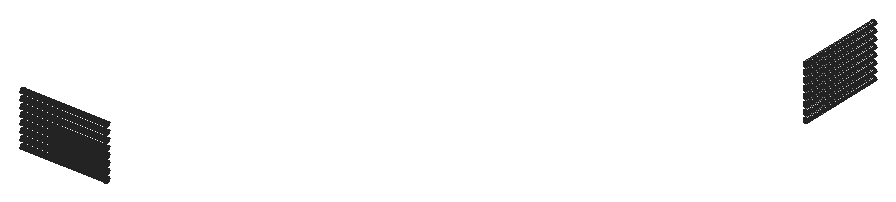
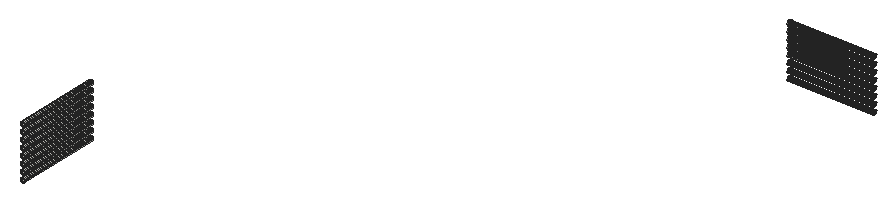
# SketchUp Ruby script. Lengths in inches.
U = 1.inch
M = Sketchup.active_model
def pt(a) = Geom::Point3d.new(a.map { |v| v * U })
def face(e, loops, mat)
  f = e.add_face(loops[0].map { |a| pt(a) })
  loops[1..].each { |l| e.add_face(l.map { |a| pt(a) }).erase! }
  f.material = f.back_material = mat if mat
  f
end
# faces: each face lists its corners as indices into pts; further lists are holes
def faces(e, pts, list, mat = nil) = list.each { |f| face(e, (f[0].is_a?(Array) ? f : [f]).map { |l| l.map { |i| pts[i] } }, mat) }
# xy, xz, yz: faces in a plane at the given z, y or x. An outline is a flat list of corners, or four numbers for a rectangle; further outlines are holes
def ring(l) = l.size == 4 ? [[l[0], l[1]], [l[2], l[1]], [l[2], l[3]], [l[0], l[3]]] : l.each_slice(2).to_a
def flat(e, list, mat, &to3) = list.each { |f| face(e, (f[0].is_a?(Array) ? f : [f]).map { |l| ring(l).map { |u, v| to3.(u, v) } }, mat) }
def xy(e, z, list, mat = nil) = flat(e, list, mat) { |x, y| [x, y, z] }
def xz(e, y, list, mat = nil) = flat(e, list, mat) { |x, z| [x, y, z] }
def yz(e, x, list, mat = nil) = flat(e, list, mat) { |y, z| [x, y, z] }
def lines(e, pts, list) = list.each { |a, b| e.add_line(pt(pts[a]), pt(pts[b])) }
# prism: a flat outline (further loops are holes) pulled along v
def prism(e, loops, v, mat = nil)
  f = face(e, loops, mat); d = Geom::Vector3d.new(v.map { |x| x * U })
  f.pushpull(f.normal.samedirection?(d) ? d.length : -d.length)
end
def box(e, o, s, mat = nil) = prism(e, [[o, [o[0] + s[0], o[1], o[2]], [o[0] + s[0], o[1] + s[1], o[2]], [o[0], o[1] + s[1], o[2]]]], [0, 0, s[2]], mat)
def at(x, y, z, deg = 0) = Geom::Transformation.translation(pt([x, y, z])) * Geom::Transformation.rotation(ORIGIN, Z_AXIS, deg.degrees)
def axes(o, x, y, z) = Geom::Transformation.new([*x, 0, *y, 0, *z, 0, *pt(o).to_a, 1])
def part(name) = M.definitions.add(name)
# library, detail: a bought-in or finely detailed component or shape, given as its bounding box
def library(name, o, s) = part(name).tap { |d| box(d.entities, o, s) }
def detail(e, o, s) = box(e.add_group.entities, o, s)
def put(e, d, t, mat = nil) = e.add_instance(d, t).tap { |i| i.material = mat if mat }
def group(e, t, mat = nil) = e.add_group.tap { |g| g.transformation = t; g.material = mat if mat }.entities
root = M.entities
p = [[922.01,48.34,1629.02],[922.01,47.38,1629.14],[778.64,47.38,1629.14],[778.64,48.34,1629.02],[922.01,49.29,1629.14],[778.64,49.29,1629.14],
  [1535.52,886.83,1629.14],[1536.47,886.83,1629.02],[1536.47,743.45,1629.02],[1535.52,743.45,1629.14],[1537.43,886.83,1629.14],[1537.43,743.45,1629.14],
  [922.01,46.5,1629.51],[778.64,46.5,1629.51],[922.01,50.18,1629.51],[778.64,50.18,1629.51],[1534.63,886.83,1629.51],[1534.63,743.45,1629.51],
  [1538.32,886.83,1629.51],[1538.32,743.45,1629.51],[922.01,45.73,1630.1],[778.64,45.73,1630.1],[922.01,50.95,1630.1],[778.64,50.95,1630.1],
  [1533.87,886.83,1630.1],[1533.87,743.45,1630.1],[1539.08,886.83,1630.1],[1539.08,743.45,1630.1],[922.01,45.15,1630.86],[778.64,45.15,1630.86],
  [922.01,51.53,1630.86],[778.64,51.53,1630.86],[1533.28,886.83,1630.86],[1533.28,743.45,1630.86],[1539.67,886.83,1630.86],[1539.67,743.45,1630.86],
  [922.01,44.78,1631.75],[778.64,44.78,1631.75],[922.01,51.9,1631.75],[778.64,51.9,1631.75],[1532.91,886.83,1631.75],[1532.91,743.45,1631.75],
  [1540.03,886.83,1631.75],[1540.03,743.45,1631.75],[922.01,44.65,1632.7],[778.64,44.65,1632.7],[922.01,52.03,1632.7],[778.64,52.03,1632.7],
  [1532.79,886.83,1632.7],[1532.79,743.45,1632.7],[1540.16,886.83,1632.7],[1540.16,743.45,1632.7],[922.01,44.78,1633.66],[778.64,44.78,1633.66],
  [922.01,51.9,1633.66],[778.64,51.9,1633.66],[1532.91,886.83,1633.66],[1532.91,743.45,1633.66],[1540.03,886.83,1633.66],[1540.03,743.45,1633.66],
  [922.01,45.15,1634.55],[778.64,45.15,1634.55],[922.01,51.53,1634.55],[778.64,51.53,1634.55],[1533.28,886.83,1634.55],[1533.28,743.45,1634.55],
  [1539.67,886.83,1634.55],[1539.67,743.45,1634.55],[922.01,45.73,1635.3125],[778.64,45.73,1635.3125],[922.01,50.95,1635.3125],[778.64,50.95,1635.3125],
  [1533.87,886.83,1635.3125],[1533.87,743.45,1635.3125],[1539.08,886.83,1635.3125],[1539.08,743.45,1635.3125],[922.01,46.5,1635.9],[778.64,46.5,1635.9],
  [922.01,50.18,1635.9],[778.64,50.18,1635.9],[1534.63,886.83,1635.9],[1534.63,743.45,1635.9],[1538.32,886.83,1635.9],[1538.32,743.45,1635.9],
  [922.01,47.38,1636.27],[778.64,47.38,1636.27],[922.01,49.29,1636.27],[778.64,49.29,1636.27],[1535.52,886.83,1636.27],[1535.52,743.45,1636.27],
  [1537.43,886.83,1636.27],[1537.43,743.45,1636.27],[922.01,48.34,1636.39],[778.64,48.34,1636.39],[1536.47,886.83,1636.39],[1536.47,743.45,1636.39],
  [922.01,48.34,1641.02],[922.01,47.38,1641.14],[778.64,47.38,1641.14],[778.64,48.34,1641.02],[922.01,49.29,1641.14],[778.64,49.29,1641.14],
  [1535.52,886.83,1641.14],[1536.47,886.83,1641.02],[1536.47,743.45,1641.02],[1535.52,743.45,1641.14],[1537.43,886.83,1641.14],[1537.43,743.45,1641.14],
  [922.01,46.5,1641.51],[778.64,46.5,1641.51],[922.01,50.18,1641.51],[778.64,50.18,1641.51],[1534.63,886.83,1641.51],[1534.63,743.45,1641.51],
  [1538.32,886.83,1641.51],[1538.32,743.45,1641.51],[922.01,45.73,1642.1],[778.64,45.73,1642.1],[922.01,50.95,1642.1],[778.64,50.95,1642.1],
  [1533.87,886.83,1642.1],[1533.87,743.45,1642.1],[1539.08,886.83,1642.1],[1539.08,743.45,1642.1],[922.01,45.15,1642.86],[778.64,45.15,1642.86],
  [922.01,51.53,1642.86],[778.64,51.53,1642.86],[1533.28,886.83,1642.86],[1533.28,743.45,1642.86],[1539.67,886.83,1642.86],[1539.67,743.45,1642.86],
  [922.01,44.78,1643.75],[778.64,44.78,1643.75],[922.01,51.9,1643.75],[778.64,51.9,1643.75],[1532.91,886.83,1643.75],[1532.91,743.45,1643.75],
  [1540.03,886.83,1643.75],[1540.03,743.45,1643.75],[922.01,44.65,1644.7],[778.64,44.65,1644.7],[922.01,52.03,1644.7],[778.64,52.03,1644.7],
  [1532.79,886.83,1644.7],[1532.79,743.45,1644.7],[1540.16,886.83,1644.7],[1540.16,743.45,1644.7],[922.01,44.78,1645.66],[778.64,44.78,1645.66],
  [922.01,51.9,1645.66],[778.64,51.9,1645.66],[1532.91,886.83,1645.66],[1532.91,743.45,1645.66],[1540.03,886.83,1645.66],[1540.03,743.45,1645.66],
  [922.01,45.15,1646.55],[778.64,45.15,1646.55],[922.01,51.53,1646.55],[778.64,51.53,1646.55],[1533.28,886.83,1646.55],[1533.28,743.45,1646.55],
  [1539.67,886.83,1646.55],[1539.67,743.45,1646.55],[922.01,45.73,1647.3125],[778.64,45.73,1647.3125],[922.01,50.95,1647.3125],[778.64,50.95,1647.3125],
  [1533.87,886.83,1647.3125],[1533.87,743.45,1647.3125],[1539.08,886.83,1647.3125],[1539.08,743.45,1647.3125],[922.01,46.5,1647.9],[778.64,46.5,1647.9],
  [922.01,50.18,1647.9],[778.64,50.18,1647.9],[1534.63,886.83,1647.9],[1534.63,743.45,1647.9],[1538.32,886.83,1647.9],[1538.32,743.45,1647.9],
  [922.01,47.38,1648.27],[778.64,47.38,1648.27],[922.01,49.29,1648.27],[778.64,49.29,1648.27],[1535.52,886.83,1648.27],[1535.52,743.45,1648.27],
  [1537.43,886.83,1648.27],[1537.43,743.45,1648.27],[922.01,48.34,1648.39],[778.64,48.34,1648.39],[1536.47,886.83,1648.39],[1536.47,743.45,1648.39],
  [922.01,48.34,1653.02],[922.01,47.38,1653.14],[778.64,47.38,1653.14],[778.64,48.34,1653.02],[922.01,49.29,1653.14],[778.64,49.29,1653.14],
  [1535.52,886.83,1653.14],[1536.47,886.83,1653.02],[1536.47,743.45,1653.02],[1535.52,743.45,1653.14],[1537.43,886.83,1653.14],[1537.43,743.45,1653.14],
  [922.01,46.5,1653.51],[778.64,46.5,1653.51],[922.01,50.18,1653.51],[778.64,50.18,1653.51],[1534.63,886.83,1653.51],[1534.63,743.45,1653.51],
  [1538.32,886.83,1653.51],[1538.32,743.45,1653.51],[922.01,45.73,1654.1],[778.64,45.73,1654.1],[922.01,50.95,1654.1],[778.64,50.95,1654.1],
  [1533.87,886.83,1654.1],[1533.87,743.45,1654.1],[1539.08,886.83,1654.1],[1539.08,743.45,1654.1],[922.01,45.15,1654.86],[778.64,45.15,1654.86],
  [922.01,51.53,1654.86],[778.64,51.53,1654.86],[1533.28,886.83,1654.86],[1533.28,743.45,1654.86],[1539.67,886.83,1654.86],[1539.67,743.45,1654.86],
  [922.01,44.78,1655.75],[778.64,44.78,1655.75],[922.01,51.9,1655.75],[778.64,51.9,1655.75],[1532.91,886.83,1655.75],[1532.91,743.45,1655.75],
  [1540.03,886.83,1655.75],[1540.03,743.45,1655.75],[922.01,44.65,1656.7],[778.64,44.65,1656.7],[922.01,52.03,1656.7],[778.64,52.03,1656.7],
  [1532.79,886.83,1656.7],[1532.79,743.45,1656.7],[1540.16,886.83,1656.7],[1540.16,743.45,1656.7],[922.01,44.78,1657.66],[778.64,44.78,1657.66],
  [922.01,51.9,1657.66],[778.64,51.9,1657.66],[1532.91,886.83,1657.66],[1532.91,743.45,1657.66],[1540.03,886.83,1657.66],[1540.03,743.45,1657.66],
  [922.01,45.15,1658.55],[778.64,45.15,1658.55],[922.01,51.53,1658.55],[778.64,51.53,1658.55],[1533.28,886.83,1658.55],[1533.28,743.45,1658.55],
  [1539.67,886.83,1658.55],[1539.67,743.45,1658.55],[922.01,45.73,1659.3125],[778.64,45.73,1659.3125],[922.01,50.95,1659.3125],[778.64,50.95,1659.3125],
  [1533.87,886.83,1659.3125],[1533.87,743.45,1659.3125],[1539.08,886.83,1659.3125],[1539.08,743.45,1659.3125],[922.01,46.5,1659.9],[778.64,46.5,1659.9],
  [922.01,50.18,1659.9],[778.64,50.18,1659.9],[1534.63,886.83,1659.9],[1534.63,743.45,1659.9],[1538.32,886.83,1659.9],[1538.32,743.45,1659.9],
  [922.01,47.38,1660.27],[778.64,47.38,1660.27],[922.01,49.29,1660.27],[778.64,49.29,1660.27],[1535.52,886.83,1660.27],[1535.52,743.45,1660.27],
  [1537.43,886.83,1660.27],[1537.43,743.45,1660.27],[922.01,48.34,1660.39],[778.64,48.34,1660.39],[1536.47,886.83,1660.39],[1536.47,743.45,1660.39],
  [922.01,48.34,1665.02],[922.01,47.38,1665.14],[778.64,47.38,1665.14],[778.64,48.34,1665.02],[922.01,49.29,1665.14],[778.64,49.29,1665.14],
  [1535.52,886.83,1665.14],[1536.47,886.83,1665.02],[1536.47,743.45,1665.02],[1535.52,743.45,1665.14],[1537.43,886.83,1665.14],[1537.43,743.45,1665.14],
  [922.01,46.5,1665.51],[778.64,46.5,1665.51],[922.01,50.18,1665.51],[778.64,50.18,1665.51],[1534.63,886.83,1665.51],[1534.63,743.45,1665.51],
  [1538.32,886.83,1665.51],[1538.32,743.45,1665.51],[922.01,45.73,1666.1],[778.64,45.73,1666.1],[922.01,50.95,1666.1],[778.64,50.95,1666.1],
  [1533.87,886.83,1666.1],[1533.87,743.45,1666.1],[1539.08,886.83,1666.1],[1539.08,743.45,1666.1],[922.01,45.15,1666.86],[778.64,45.15,1666.86],
  [922.01,51.53,1666.86],[778.64,51.53,1666.86],[1533.28,886.83,1666.86],[1533.28,743.45,1666.86],[1539.67,886.83,1666.86],[1539.67,743.45,1666.86],
  [922.01,44.78,1667.75],[778.64,44.78,1667.75],[922.01,51.9,1667.75],[778.64,51.9,1667.75],[1532.91,886.83,1667.75],[1532.91,743.45,1667.75],
  [1540.03,886.83,1667.75],[1540.03,743.45,1667.75],[922.01,44.65,1668.7],[778.64,44.65,1668.7],[922.01,52.03,1668.7],[778.64,52.03,1668.7],
  [1532.79,886.83,1668.7],[1532.79,743.45,1668.7],[1540.16,886.83,1668.7],[1540.16,743.45,1668.7],[922.01,44.78,1669.66],[778.64,44.78,1669.66],
  [922.01,51.9,1669.66],[778.64,51.9,1669.66],[1532.91,886.83,1669.66],[1532.91,743.45,1669.66],[1540.03,886.83,1669.66],[1540.03,743.45,1669.66],
  [922.01,45.15,1670.55],[778.64,45.15,1670.55],[922.01,51.53,1670.55],[778.64,51.53,1670.55],[1533.28,886.83,1670.55],[1533.28,743.45,1670.55],
  [1539.67,886.83,1670.55],[1539.67,743.45,1670.55],[922.01,45.73,1671.3125],[778.64,45.73,1671.3125],[922.01,50.95,1671.3125],[778.64,50.95,1671.3125],
  [1533.87,886.83,1671.3125],[1533.87,743.45,1671.3125],[1539.08,886.83,1671.3125],[1539.08,743.45,1671.3125],[922.01,46.5,1671.9],[778.64,46.5,1671.9],
  [922.01,50.18,1671.9],[778.64,50.18,1671.9],[1534.63,886.83,1671.9],[1534.63,743.45,1671.9],[1538.32,886.83,1671.9],[1538.32,743.45,1671.9],
  [922.01,47.38,1672.27],[778.64,47.38,1672.27],[922.01,49.29,1672.27],[778.64,49.29,1672.27],[1535.52,886.83,1672.27],[1535.52,743.45,1672.27],
  [1537.43,886.83,1672.27],[1537.43,743.45,1672.27],[922.01,48.34,1672.39],[778.64,48.34,1672.39],[1536.47,886.83,1672.39],[1536.47,743.45,1672.39],
  [922.01,48.34,1677.02],[922.01,47.38,1677.14],[778.64,47.38,1677.14],[778.64,48.34,1677.02],[922.01,49.29,1677.14],[778.64,49.29,1677.14],
  [1535.52,886.83,1677.14],[1536.47,886.83,1677.02],[1536.47,743.45,1677.02],[1535.52,743.45,1677.14],[1537.43,886.83,1677.14],[1537.43,743.45,1677.14],
  [922.01,46.5,1677.51],[778.64,46.5,1677.51],[922.01,50.18,1677.51],[778.64,50.18,1677.51],[1534.63,886.83,1677.51],[1534.63,743.45,1677.51],
  [1538.32,886.83,1677.51],[1538.32,743.45,1677.51],[922.01,45.73,1678.1],[778.64,45.73,1678.1],[922.01,50.95,1678.1],[778.64,50.95,1678.1],
  [1533.87,886.83,1678.1],[1533.87,743.45,1678.1],[1539.08,886.83,1678.1],[1539.08,743.45,1678.1],[922.01,45.15,1678.86],[778.64,45.15,1678.86],
  [922.01,51.53,1678.86],[778.64,51.53,1678.86],[1533.28,886.83,1678.86],[1533.28,743.45,1678.86],[1539.67,886.83,1678.86],[1539.67,743.45,1678.86],
  [922.01,44.78,1679.75],[778.64,44.78,1679.75],[922.01,51.9,1679.75],[778.64,51.9,1679.75],[1532.91,886.83,1679.75],[1532.91,743.45,1679.75],
  [1540.03,886.83,1679.75],[1540.03,743.45,1679.75],[922.01,44.65,1680.7],[778.64,44.65,1680.7],[922.01,52.03,1680.7],[778.64,52.03,1680.7],
  [1532.79,886.83,1680.7],[1532.79,743.45,1680.7],[1540.16,886.83,1680.7],[1540.16,743.45,1680.7],[922.01,44.78,1681.66],[778.64,44.78,1681.66],
  [922.01,51.9,1681.66],[778.64,51.9,1681.66],[1532.91,886.83,1681.66],[1532.91,743.45,1681.66],[1540.03,886.83,1681.66],[1540.03,743.45,1681.66],
  [922.01,45.15,1682.55],[778.64,45.15,1682.55],[922.01,51.53,1682.55],[778.64,51.53,1682.55],[1533.28,886.83,1682.55],[1533.28,743.45,1682.55],
  [1539.67,886.83,1682.55],[1539.67,743.45,1682.55],[922.01,45.73,1683.3125],[778.64,45.73,1683.3125],[922.01,50.95,1683.3125],[778.64,50.95,1683.3125],
  [1533.87,886.83,1683.3125],[1533.87,743.45,1683.3125],[1539.08,886.83,1683.3125],[1539.08,743.45,1683.3125],[922.01,46.5,1683.9],[778.64,46.5,1683.9],
  [922.01,50.18,1683.9],[778.64,50.18,1683.9],[1534.63,886.83,1683.9],[1534.63,743.45,1683.9],[1538.32,886.83,1683.9],[1538.32,743.45,1683.9],
  [922.01,47.38,1684.27],[778.64,47.38,1684.27],[922.01,49.29,1684.27],[778.64,49.29,1684.27],[1535.52,886.83,1684.27],[1535.52,743.45,1684.27],
  [1537.43,886.83,1684.27],[1537.43,743.45,1684.27],[922.01,48.34,1684.39],[778.64,48.34,1684.39],[1536.47,886.83,1684.39],[1536.47,743.45,1684.39],
  [922.01,48.34,1689.02],[922.01,47.38,1689.14],[778.64,47.38,1689.14],[778.64,48.34,1689.02],[922.01,49.29,1689.14],[778.64,49.29,1689.14],
  [1535.52,886.83,1689.14],[1536.47,886.83,1689.02],[1536.47,743.45,1689.02],[1535.52,743.45,1689.14],[1537.43,886.83,1689.14],[1537.43,743.45,1689.14],
  [922.01,46.5,1689.51],[778.64,46.5,1689.51],[922.01,50.18,1689.51],[778.64,50.18,1689.51],[1534.63,886.83,1689.51],[1534.63,743.45,1689.51],
  [1538.32,886.83,1689.51],[1538.32,743.45,1689.51],[922.01,45.73,1690.1],[778.64,45.73,1690.1],[922.01,50.95,1690.1],[778.64,50.95,1690.1],
  [1533.87,886.83,1690.1],[1533.87,743.45,1690.1],[1539.08,886.83,1690.1],[1539.08,743.45,1690.1],[922.01,45.15,1690.86],[778.64,45.15,1690.86],
  [922.01,51.53,1690.86],[778.64,51.53,1690.86],[1533.28,886.83,1690.86],[1533.28,743.45,1690.86],[1539.67,886.83,1690.86],[1539.67,743.45,1690.86],
  [922.01,44.78,1691.75],[778.64,44.78,1691.75],[922.01,51.9,1691.75],[778.64,51.9,1691.75],[1532.91,886.83,1691.75],[1532.91,743.45,1691.75],
  [1540.03,886.83,1691.75],[1540.03,743.45,1691.75],[922.01,44.65,1692.7],[778.64,44.65,1692.7],[922.01,52.03,1692.7],[778.64,52.03,1692.7],
  [1532.79,886.83,1692.7],[1532.79,743.45,1692.7],[1540.16,886.83,1692.7],[1540.16,743.45,1692.7],[922.01,44.78,1693.66],[778.64,44.78,1693.66],
  [922.01,51.9,1693.66],[778.64,51.9,1693.66],[1532.91,886.83,1693.66],[1532.91,743.45,1693.66],[1540.03,886.83,1693.66],[1540.03,743.45,1693.66],
  [922.01,45.15,1694.55],[778.64,45.15,1694.55],[922.01,51.53,1694.55],[778.64,51.53,1694.55],[1533.28,886.83,1694.55],[1533.28,743.45,1694.55],
  [1539.67,886.83,1694.55],[1539.67,743.45,1694.55],[922.01,45.73,1695.3125],[778.64,45.73,1695.3125],[922.01,50.95,1695.3125],[778.64,50.95,1695.3125],
  [1533.87,886.83,1695.3125],[1533.87,743.45,1695.3125],[1539.08,886.83,1695.3125],[1539.08,743.45,1695.3125],[922.01,46.5,1695.9],[778.64,46.5,1695.9],
  [922.01,50.18,1695.9],[778.64,50.18,1695.9],[1534.63,886.83,1695.9],[1534.63,743.45,1695.9],[1538.32,886.83,1695.9],[1538.32,743.45,1695.9],
  [922.01,47.38,1696.27],[778.64,47.38,1696.27],[922.01,49.29,1696.27],[778.64,49.29,1696.27],[1535.52,886.83,1696.27],[1535.52,743.45,1696.27],
  [1537.43,886.83,1696.27],[1537.43,743.45,1696.27],[922.01,48.34,1696.39],[778.64,48.34,1696.39],[1536.47,886.83,1696.39],[1536.47,743.45,1696.39],
  [922.01,48.34,1701.02],[922.01,47.38,1701.14],[778.64,47.38,1701.14],[778.64,48.34,1701.02],[922.01,49.29,1701.14],[778.64,49.29,1701.14],
  [1535.52,886.83,1701.14],[1536.47,886.83,1701.02],[1536.47,743.45,1701.02],[1535.52,743.45,1701.14],[1537.43,886.83,1701.14],[1537.43,743.45,1701.14],
  [922.01,46.5,1701.51],[778.64,46.5,1701.51],[922.01,50.18,1701.51],[778.64,50.18,1701.51],[1534.63,886.83,1701.51],[1534.63,743.45,1701.51],
  [1538.32,886.83,1701.51],[1538.32,743.45,1701.51],[922.01,45.73,1702.1],[778.64,45.73,1702.1],[922.01,50.95,1702.1],[778.64,50.95,1702.1],
  [1533.87,886.83,1702.1],[1533.87,743.45,1702.1],[1539.08,886.83,1702.1],[1539.08,743.45,1702.1],[922.01,45.15,1702.86],[778.64,45.15,1702.86],
  [922.01,51.53,1702.86],[778.64,51.53,1702.86],[1533.28,886.83,1702.86],[1533.28,743.45,1702.86],[1539.67,886.83,1702.86],[1539.67,743.45,1702.86],
  [922.01,44.78,1703.75],[778.64,44.78,1703.75],[922.01,51.9,1703.75],[778.64,51.9,1703.75],[1532.91,886.83,1703.75],[1532.91,743.45,1703.75],
  [1540.03,886.83,1703.75],[1540.03,743.45,1703.75],[922.01,44.65,1704.7],[778.64,44.65,1704.7],[922.01,52.03,1704.7],[778.64,52.03,1704.7],
  [1532.79,886.83,1704.7],[1532.79,743.45,1704.7],[1540.16,886.83,1704.7],[1540.16,743.45,1704.7],[922.01,44.78,1705.66],[778.64,44.78,1705.66],
  [922.01,51.9,1705.66],[778.64,51.9,1705.66],[1532.91,886.83,1705.66],[1532.91,743.45,1705.66],[1540.03,886.83,1705.66],[1540.03,743.45,1705.66],
  [922.01,45.15,1706.55],[778.64,45.15,1706.55],[922.01,51.53,1706.55],[778.64,51.53,1706.55],[1533.28,886.83,1706.55],[1533.28,743.45,1706.55],
  [1539.67,886.83,1706.55],[1539.67,743.45,1706.55],[922.01,45.73,1707.3125],[778.64,45.73,1707.3125],[922.01,50.95,1707.3125],[778.64,50.95,1707.3125],
  [1533.87,886.83,1707.3125],[1533.87,743.45,1707.3125],[1539.08,886.83,1707.3125],[1539.08,743.45,1707.3125],[922.01,46.5,1707.9],[778.64,46.5,1707.9],
  [922.01,50.18,1707.9],[778.64,50.18,1707.9],[1534.63,886.83,1707.9],[1534.63,743.45,1707.9],[1538.32,886.83,1707.9],[1538.32,743.45,1707.9],
  [922.01,47.38,1708.27],[778.64,47.38,1708.27],[922.01,49.29,1708.27],[778.64,49.29,1708.27],[1535.52,886.83,1708.27],[1535.52,743.45,1708.27],
  [1537.43,886.83,1708.27],[1537.43,743.45,1708.27],[922.01,48.34,1708.39],[778.64,48.34,1708.39],[1536.47,886.83,1708.39],[1536.47,743.45,1708.39],
  [922.01,48.34,1713.02],[922.01,47.38,1713.14],[778.64,47.38,1713.14],[778.64,48.34,1713.02],[922.01,49.29,1713.14],[778.64,49.29,1713.14],
  [1535.52,886.83,1713.14],[1536.47,886.83,1713.02],[1536.47,743.45,1713.02],[1535.52,743.45,1713.14],[1537.43,886.83,1713.14],[1537.43,743.45,1713.14],
  [922.01,46.5,1713.51],[778.64,46.5,1713.51],[922.01,50.18,1713.51],[778.64,50.18,1713.51],[1534.63,886.83,1713.51],[1534.63,743.45,1713.51],
  [1538.32,886.83,1713.51],[1538.32,743.45,1713.51],[922.01,45.73,1714.1],[778.64,45.73,1714.1],[922.01,50.95,1714.1],[778.64,50.95,1714.1],
  [1533.87,886.83,1714.1],[1533.87,743.45,1714.1],[1539.08,886.83,1714.1],[1539.08,743.45,1714.1],[922.01,45.15,1714.86],[778.64,45.15,1714.86],
  [922.01,51.53,1714.86],[778.64,51.53,1714.86],[1533.28,886.83,1714.86],[1533.28,743.45,1714.86],[1539.67,886.83,1714.86],[1539.67,743.45,1714.86],
  [922.01,44.78,1715.75],[778.64,44.78,1715.75],[922.01,51.9,1715.75],[778.64,51.9,1715.75],[1532.91,886.83,1715.75],[1532.91,743.45,1715.75],
  [1540.03,886.83,1715.75],[1540.03,743.45,1715.75],[922.01,44.65,1716.7],[778.64,44.65,1716.7],[922.01,52.03,1716.7],[778.64,52.03,1716.7],
  [1532.79,886.83,1716.7],[1532.79,743.45,1716.7],[1540.16,886.83,1716.7],[1540.16,743.45,1716.7],[922.01,44.78,1717.66],[778.64,44.78,1717.66],
  [922.01,51.9,1717.66],[778.64,51.9,1717.66],[1532.91,886.83,1717.66],[1532.91,743.45,1717.66],[1540.03,886.83,1717.66],[1540.03,743.45,1717.66],
  [922.01,45.15,1718.55],[778.64,45.15,1718.55],[922.01,51.53,1718.55],[778.64,51.53,1718.55],[1533.28,886.83,1718.55],[1533.28,743.45,1718.55],
  [1539.67,886.83,1718.55],[1539.67,743.45,1718.55],[922.01,45.73,1719.3125],[778.64,45.73,1719.3125],[922.01,50.95,1719.3125],[778.64,50.95,1719.3125],
  [1533.87,886.83,1719.3125],[1533.87,743.45,1719.3125],[1539.08,886.83,1719.3125],[1539.08,743.45,1719.3125],[922.01,46.5,1719.9],[778.64,46.5,1719.9],
  [922.01,50.18,1719.9],[778.64,50.18,1719.9],[1534.63,886.83,1719.9],[1534.63,743.45,1719.9],[1538.32,886.83,1719.9],[1538.32,743.45,1719.9],
  [922.01,47.38,1720.27],[778.64,47.38,1720.27],[922.01,49.29,1720.27],[778.64,49.29,1720.27],[1535.52,886.83,1720.27],[1535.52,743.45,1720.27],
  [1537.43,886.83,1720.27],[1537.43,743.45,1720.27],[922.01,48.34,1720.39],[778.64,48.34,1720.39],[1536.47,886.83,1720.39],[1536.47,743.45,1720.39]]
faces(root,p,[[0,1,2,3],[4,0,3,5],[6,7,8,9],[7,10,11,8],[1,12,13,2],[14,4,5,15],[16,6,9,17],[10,18,19,11],
  [12,20,21,13],[22,14,15,23],[24,16,17,25],[18,26,27,19],[20,28,29,21],[30,22,23,31],[32,24,25,33],[26,34,35,27],
  [28,36,37,29],[38,30,31,39],[40,32,33,41],[34,42,43,35],[36,44,45,37],[46,38,39,47],[48,40,41,49],[42,50,51,43],
  [44,52,53,45],[54,46,47,55],[56,48,49,57],[50,58,59,51],[52,60,61,53],[62,54,55,63],[64,56,57,65],[58,66,67,59],
  [60,68,69,61],[70,62,63,71],[72,64,65,73],[66,74,75,67],[68,76,77,69],[78,70,71,79],[80,72,73,81],[74,82,83,75],
  [76,84,85,77],[86,78,79,87],[88,80,81,89],[82,90,91,83],[84,92,93,85],[92,86,87,93],[94,88,89,95],[90,94,95,91],
  [96,97,98,99],[100,96,99,101],[102,103,104,105],[103,106,107,104],[97,108,109,98],[110,100,101,111],[112,102,105,113],[106,114,115,107],
  [108,116,117,109],[118,110,111,119],[120,112,113,121],[114,122,123,115],[116,124,125,117],[126,118,119,127],[128,120,121,129],[122,130,131,123],
  [124,132,133,125],[134,126,127,135],[136,128,129,137],[130,138,139,131],[132,140,141,133],[142,134,135,143],[144,136,137,145],[138,146,147,139],
  [140,148,149,141],[150,142,143,151],[152,144,145,153],[146,154,155,147],[148,156,157,149],[158,150,151,159],[160,152,153,161],[154,162,163,155],
  [156,164,165,157],[166,158,159,167],[168,160,161,169],[162,170,171,163],[164,172,173,165],[174,166,167,175],[176,168,169,177],[170,178,179,171],
  [172,180,181,173],[182,174,175,183],[184,176,177,185],[178,186,187,179],[180,188,189,181],[188,182,183,189],[190,184,185,191],[186,190,191,187],
  [192,193,194,195],[196,192,195,197],[198,199,200,201],[199,202,203,200],[193,204,205,194],[206,196,197,207],[208,198,201,209],[202,210,211,203],
  [204,212,213,205],[214,206,207,215],[216,208,209,217],[210,218,219,211],[212,220,221,213],[222,214,215,223],[224,216,217,225],[218,226,227,219],
  [220,228,229,221],[230,222,223,231],[232,224,225,233],[226,234,235,227],[228,236,237,229],[238,230,231,239],[240,232,233,241],[234,242,243,235],
  [236,244,245,237],[246,238,239,247],[248,240,241,249],[242,250,251,243],[244,252,253,245],[254,246,247,255],[256,248,249,257],[250,258,259,251],
  [252,260,261,253],[262,254,255,263],[264,256,257,265],[258,266,267,259],[260,268,269,261],[270,262,263,271],[272,264,265,273],[266,274,275,267],
  [268,276,277,269],[278,270,271,279],[280,272,273,281],[274,282,283,275],[276,284,285,277],[284,278,279,285],[286,280,281,287],[282,286,287,283],
  [288,289,290,291],[292,288,291,293],[294,295,296,297],[295,298,299,296],[289,300,301,290],[302,292,293,303],[304,294,297,305],[298,306,307,299],
  [300,308,309,301],[310,302,303,311],[312,304,305,313],[306,314,315,307],[308,316,317,309],[318,310,311,319],[320,312,313,321],[314,322,323,315],
  [316,324,325,317],[326,318,319,327],[328,320,321,329],[322,330,331,323],[324,332,333,325],[334,326,327,335],[336,328,329,337],[330,338,339,331],
  [332,340,341,333],[342,334,335,343],[344,336,337,345],[338,346,347,339],[340,348,349,341],[350,342,343,351],[352,344,345,353],[346,354,355,347],
  [348,356,357,349],[358,350,351,359],[360,352,353,361],[354,362,363,355],[356,364,365,357],[366,358,359,367],[368,360,361,369],[362,370,371,363],
  [364,372,373,365],[374,366,367,375],[376,368,369,377],[370,378,379,371],[372,380,381,373],[380,374,375,381],[382,376,377,383],[378,382,383,379],
  [384,385,386,387],[388,384,387,389],[390,391,392,393],[391,394,395,392],[385,396,397,386],[398,388,389,399],[400,390,393,401],[394,402,403,395],
  [396,404,405,397],[406,398,399,407],[408,400,401,409],[402,410,411,403],[404,412,413,405],[414,406,407,415],[416,408,409,417],[410,418,419,411],
  [412,420,421,413],[422,414,415,423],[424,416,417,425],[418,426,427,419],[420,428,429,421],[430,422,423,431],[432,424,425,433],[426,434,435,427],
  [428,436,437,429],[438,430,431,439],[440,432,433,441],[434,442,443,435],[436,444,445,437],[446,438,439,447],[448,440,441,449],[442,450,451,443],
  [444,452,453,445],[454,446,447,455],[456,448,449,457],[450,458,459,451],[452,460,461,453],[462,454,455,463],[464,456,457,465],[458,466,467,459],
  [460,468,469,461],[470,462,463,471],[472,464,465,473],[466,474,475,467],[468,476,477,469],[476,470,471,477],[478,472,473,479],[474,478,479,475],
  [480,481,482,483],[484,480,483,485],[486,487,488,489],[487,490,491,488],[481,492,493,482],[494,484,485,495],[496,486,489,497],[490,498,499,491],
  [492,500,501,493],[502,494,495,503],[504,496,497,505],[498,506,507,499],[500,508,509,501],[510,502,503,511],[512,504,505,513],[506,514,515,507],
  [508,516,517,509],[518,510,511,519],[520,512,513,521],[514,522,523,515],[516,524,525,517],[526,518,519,527],[528,520,521,529],[522,530,531,523],
  [524,532,533,525],[534,526,527,535],[536,528,529,537],[530,538,539,531],[532,540,541,533],[542,534,535,543],[544,536,537,545],[538,546,547,539],
  [540,548,549,541],[550,542,543,551],[552,544,545,553],[546,554,555,547],[548,556,557,549],[558,550,551,559],[560,552,553,561],[554,562,563,555],
  [556,564,565,557],[566,558,559,567],[568,560,561,569],[562,570,571,563],[564,572,573,565],[572,566,567,573],[574,568,569,575],[570,574,575,571],
  [576,577,578,579],[580,576,579,581],[582,583,584,585],[583,586,587,584],[577,588,589,578],[590,580,581,591],[592,582,585,593],[586,594,595,587],
  [588,596,597,589],[598,590,591,599],[600,592,593,601],[594,602,603,595],[596,604,605,597],[606,598,599,607],[608,600,601,609],[602,610,611,603],
  [604,612,613,605],[614,606,607,615],[616,608,609,617],[610,618,619,611],[612,620,621,613],[622,614,615,623],[624,616,617,625],[618,626,627,619],
  [620,628,629,621],[630,622,623,631],[632,624,625,633],[626,634,635,627],[628,636,637,629],[638,630,631,639],[640,632,633,641],[634,642,643,635],
  [636,644,645,637],[646,638,639,647],[648,640,641,649],[642,650,651,643],[644,652,653,645],[654,646,647,655],[656,648,649,657],[650,658,659,651],
  [652,660,661,653],[662,654,655,663],[664,656,657,665],[658,666,667,659],[660,668,669,661],[668,662,663,669],[670,664,665,671],[666,670,671,667],
  [672,673,674,675],[676,672,675,677],[678,679,680,681],[679,682,683,680],[673,684,685,674],[686,676,677,687],[688,678,681,689],[682,690,691,683],
  [684,692,693,685],[694,686,687,695],[696,688,689,697],[690,698,699,691],[692,700,701,693],[702,694,695,703],[704,696,697,705],[698,706,707,699],
  [700,708,709,701],[710,702,703,711],[712,704,705,713],[706,714,715,707],[708,716,717,709],[718,710,711,719],[720,712,713,721],[714,722,723,715],
  [716,724,725,717],[726,718,719,727],[728,720,721,729],[722,730,731,723],[724,732,733,725],[734,726,727,735],[736,728,729,737],[730,738,739,731],
  [732,740,741,733],[742,734,735,743],[744,736,737,745],[738,746,747,739],[740,748,749,741],[750,742,743,751],[752,744,745,753],[746,754,755,747],
  [748,756,757,749],[758,750,751,759],[760,752,753,761],[754,762,763,755],[756,764,765,757],[764,758,759,765],[766,760,761,767],[762,766,767,763]])
